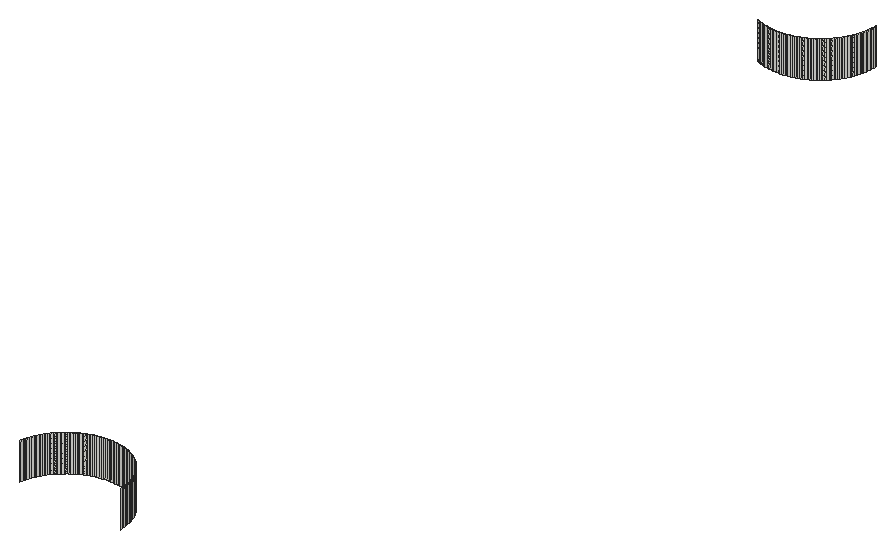
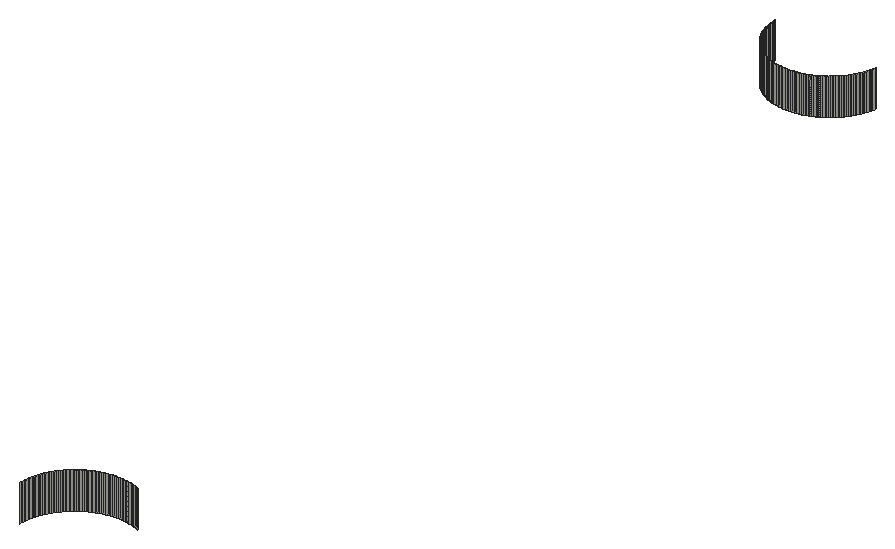
# SketchUp Ruby script. Lengths in inches.
U = 1.inch
M = Sketchup.active_model
def pt(a) = Geom::Point3d.new(a.map { |v| v * U })
def face(e, loops, mat)
  f = e.add_face(loops[0].map { |a| pt(a) })
  loops[1..].each { |l| e.add_face(l.map { |a| pt(a) }).erase! }
  f.material = f.back_material = mat if mat
  f
end
# faces: each face lists its corners as indices into pts; further lists are holes
def faces(e, pts, list, mat = nil) = list.each { |f| face(e, (f[0].is_a?(Array) ? f : [f]).map { |l| l.map { |i| pts[i] } }, mat) }
# xy, xz, yz: faces in a plane at the given z, y or x. An outline is a flat list of corners, or four numbers for a rectangle; further outlines are holes
def ring(l) = l.size == 4 ? [[l[0], l[1]], [l[2], l[1]], [l[2], l[3]], [l[0], l[3]]] : l.each_slice(2).to_a
def flat(e, list, mat, &to3) = list.each { |f| face(e, (f[0].is_a?(Array) ? f : [f]).map { |l| ring(l).map { |u, v| to3.(u, v) } }, mat) }
def xy(e, z, list, mat = nil) = flat(e, list, mat) { |x, y| [x, y, z] }
def xz(e, y, list, mat = nil) = flat(e, list, mat) { |x, z| [x, y, z] }
def yz(e, x, list, mat = nil) = flat(e, list, mat) { |y, z| [x, y, z] }
def lines(e, pts, list) = list.each { |a, b| e.add_line(pt(pts[a]), pt(pts[b])) }
# prism: a flat outline (further loops are holes) pulled along v
def prism(e, loops, v, mat = nil)
  f = face(e, loops, mat); d = Geom::Vector3d.new(v.map { |x| x * U })
  f.pushpull(f.normal.samedirection?(d) ? d.length : -d.length)
end
def box(e, o, s, mat = nil) = prism(e, [[o, [o[0] + s[0], o[1], o[2]], [o[0] + s[0], o[1] + s[1], o[2]], [o[0], o[1] + s[1], o[2]]]], [0, 0, s[2]], mat)
def at(x, y, z, deg = 0) = Geom::Transformation.translation(pt([x, y, z])) * Geom::Transformation.rotation(ORIGIN, Z_AXIS, deg.degrees)
def axes(o, x, y, z) = Geom::Transformation.new([*x, 0, *y, 0, *z, 0, *pt(o).to_a, 1])
def part(name) = M.definitions.add(name)
# library, detail: a bought-in or finely detailed component or shape, given as its bounding box
def library(name, o, s) = part(name).tap { |d| box(d.entities, o, s) }
def detail(e, o, s) = box(e.add_group.entities, o, s)
def put(e, d, t, mat = nil) = e.add_instance(d, t).tap { |i| i.material = mat if mat }
def group(e, t, mat = nil) = e.add_group.tap { |g| g.transformation = t; g.material = mat if mat }.entities
root = M.entities
xz(root,27,[[156.34,108,156.42,110],[156.42,108,156.5,110],[156.5,108,156.58,110],[156.58,108,156.66,110]])
xz(root,72.5,[[156.34,108,156.42,110],[156.42,108,156.5,110],[156.5,108,156.58,110],[156.58,108,156.66,110]])
yz(root,159.5,[[24,108,24.08,110],[24.08,108,24.16,110],[75.34,108,75.42,110],[75.42,108,75.5,110]])
p = [[159.48,24.3125,108],[159.49,24.24,108],[159.49,24.24,110],[159.48,24.3125,110],[159.5,24.16,108],[159.5,24.16,110],
  [159.47,24.39,108],[159.47,24.39,110],[159.46,24.47,108],[159.46,24.47,110],[153.55,24.55,108],[153.57,24.625,108],
  [153.57,24.625,110],[153.55,24.55,110],[159.43,24.625,108],[159.45,24.55,108],[159.45,24.55,110],[159.43,24.625,110],
  [153.58,24.7,108],[153.58,24.7,110],[159.42,24.7,108],[159.42,24.7,110],[153.6,24.78,108],[153.6,24.78,110],
  [159.4,24.78,108],[159.4,24.78,110],[153.625,24.85,108],[153.625,24.85,110],[159.375,24.85,108],[159.375,24.85,110],
  [153.65,24.93,108],[153.65,24.93,110],[153.67,25,108],[153.67,25,110],[159.33,25,108],[159.35,24.93,108],
  [159.35,24.93,110],[159.33,25,110],[153.7,25.08,108],[153.7,25.08,110],[159.3,25.08,108],[159.3,25.08,110],
  [153.73,25.15,108],[153.73,25.15,110],[153.76,25.22,108],[153.76,25.22,110],[159.24,25.22,108],[159.27,25.15,108],
  [159.27,25.15,110],[159.24,25.22,110],[153.79,25.29,108],[153.79,25.29,110],[159.21,25.29,108],[159.21,25.29,110],
  [153.83,25.36,108],[153.83,25.36,110],[159.17,25.36,108],[159.17,25.36,110],[153.86,25.43,108],[153.86,25.43,110],
  [153.9,25.5,108],[153.9,25.5,110],[159.1,25.5,108],[159.14,25.43,108],[159.14,25.43,110],[159.1,25.5,110],
  [153.94,25.57,108],[153.94,25.57,110],[159.06,25.57,108],[159.06,25.57,110],[153.98,25.63,108],[153.98,25.63,110],
  [154.03,25.7,108],[154.03,25.7,110],[158.97,25.7,108],[159.02,25.63,108],[159.02,25.63,110],[158.97,25.7,110],
  [154.07,25.76,108],[154.07,25.76,110],[158.93,25.76,108],[158.93,25.76,110],[154.12,25.83,108],[154.12,25.83,110],
  [154.17,25.89,108],[154.17,25.89,110],[158.83,25.89,108],[158.88,25.83,108],[158.88,25.83,110],[158.83,25.89,110],
  [154.22,25.95,108],[154.22,25.95,110],[154.27,26.01,108],[154.27,26.01,110],[158.73,26.01,108],[158.78,25.95,108],
  [158.78,25.95,110],[158.73,26.01,110],[154.32,26.07,108],[154.32,26.07,110],[158.68,26.07,108],[158.68,26.07,110],
  [154.38,26.12,108],[154.38,26.12,110],[154.43,26.18,108],[154.43,26.18,110],[158.57,26.18,108],[158.62,26.12,108],
  [158.62,26.12,110],[158.57,26.18,110],[154.49,26.23,108],[154.49,26.23,110],[154.55,26.28,108],[154.55,26.28,110],
  [158.45,26.28,108],[158.51,26.23,108],[158.51,26.23,110],[158.45,26.28,110],[154.61,26.33,108],[154.61,26.33,110],
  [154.67,26.38,108],[154.67,26.38,110],[158.33,26.38,108],[158.39,26.33,108],[158.39,26.33,110],[158.33,26.38,110],
  [154.74,26.43,108],[154.74,26.43,110],[154.8,26.47,108],[154.8,26.47,110],[158.2,26.47,108],[158.26,26.43,108],
  [158.26,26.43,110],[158.2,26.47,110],[154.87,26.52,108],[154.87,26.52,110],[154.93,26.56,108],[154.93,26.56,110],
  [158.07,26.56,108],[158.13,26.52,108],[158.13,26.52,110],[158.07,26.56,110],[155,26.6,108],[155,26.6,110],
  [155.07,26.64,108],[155.07,26.64,110],[155.14,26.67,108],[155.14,26.67,110],[157.86,26.67,108],[157.93,26.64,108],
  [157.93,26.64,110],[157.86,26.67,110],[158,26.6,108],[158,26.6,110],[155.21,26.71,108],[155.21,26.71,110],
  [155.28,26.74,108],[155.28,26.74,110],[155.35,26.77,108],[155.35,26.77,110],[157.65,26.77,108],[157.72,26.74,108],
  [157.72,26.74,110],[157.65,26.77,110],[157.79,26.71,108],[157.79,26.71,110],[155.42,26.8,108],[155.42,26.8,110],
  [155.5,26.83,108],[155.5,26.83,110],[155.57,26.85,108],[155.57,26.85,110],[157.43,26.85,108],[157.5,26.83,108],
  [157.5,26.83,110],[157.43,26.85,110],[157.58,26.8,108],[157.58,26.8,110],[155.65,26.875,108],[155.65,26.875,110],
  [155.72,26.9,108],[155.72,26.9,110],[155.8,26.92,108],[155.8,26.92,110],[155.875,26.93,108],[155.875,26.93,110],
  [155.95,26.95,108],[155.95,26.95,110],[156.03,26.96,108],[156.03,26.96,110],[156.97,26.96,108],[157.05,26.95,108],
  [157.05,26.95,110],[156.97,26.96,110],[157.125,26.93,108],[157.125,26.93,110],[157.2,26.92,108],[157.2,26.92,110],
  [157.28,26.9,108],[157.28,26.9,110],[157.35,26.875,108],[157.35,26.875,110],[156.11,26.97,108],[156.11,26.97,110],
  [156.1875,26.98,108],[156.1875,26.98,110],[156.26,26.99,108],[156.26,26.99,110],[156.34,27,108],[156.34,27,110],
  [156.66,27,108],[156.74,26.99,108],[156.74,26.99,110],[156.66,27,110],[156.8125,26.98,108],[156.8125,26.98,110],
  [156.89,26.97,108],[156.89,26.97,110],[156.11,72.53,108],[156.03,72.54,108],[156.03,72.54,110],[156.11,72.53,110],
  [155.95,72.55,108],[155.95,72.55,110],[156.1875,72.52,108],[156.1875,72.52,110],[156.26,72.51,108],[156.26,72.51,110],
  [156.34,72.5,108],[156.34,72.5,110],[156.8125,72.52,108],[156.74,72.51,108],[156.74,72.51,110],[156.8125,72.52,110],
  [156.66,72.5,108],[156.66,72.5,110],[156.89,72.53,108],[156.89,72.53,110],[156.97,72.54,108],[156.97,72.54,110],
  [157.05,72.55,108],[157.05,72.55,110],[155.57,72.65,108],[155.5,72.67,108],[155.5,72.67,110],[155.57,72.65,110],
  [155.72,72.6,108],[155.65,72.625,108],[155.65,72.625,110],[155.72,72.6,110],[155.8,72.58,108],[155.8,72.58,110],
  [155.875,72.57,108],[155.875,72.57,110],[157.125,72.57,108],[157.125,72.57,110],[157.2,72.58,108],[157.2,72.58,110],
  [157.28,72.6,108],[157.28,72.6,110],[157.35,72.625,108],[157.35,72.625,110],[157.5,72.67,108],[157.43,72.65,108],
  [157.43,72.65,110],[157.5,72.67,110],[155.35,72.73,108],[155.28,72.76,108],[155.28,72.76,110],[155.35,72.73,110],
  [155.42,72.7,108],[155.42,72.7,110],[157.58,72.7,108],[157.58,72.7,110],[157.72,72.76,108],[157.65,72.73,108],
  [157.65,72.73,110],[157.72,72.76,110],[157.79,72.79,108],[157.79,72.79,110],[157.86,72.83,108],[157.86,72.83,110],
  [157.93,72.86,108],[157.93,72.86,110],[158,72.9,108],[158,72.9,110],[158.07,72.94,108],[158.07,72.94,110],
  [158.13,72.98,108],[158.13,72.98,110],[158.2,73.03,108],[158.2,73.03,110],[158.26,73.07,108],[158.26,73.07,110],
  [158.39,73.17,108],[158.33,73.12,108],[158.33,73.12,110],[158.39,73.17,110],[158.51,73.27,108],[158.45,73.22,108],
  [158.45,73.22,110],[158.51,73.27,110],[158.57,73.32,108],[158.57,73.32,110],[158.62,73.38,108],[158.62,73.38,110],
  [158.68,73.43,108],[158.68,73.43,110],[158.73,73.49,108],[158.73,73.49,110],[158.78,73.55,108],[158.78,73.55,110],
  [158.88,73.67,108],[158.83,73.61,108],[158.83,73.61,110],[158.88,73.67,110],[158.97,73.8,108],[158.93,73.74,108],
  [158.93,73.74,110],[158.97,73.8,110],[159.02,73.87,108],[159.02,73.87,110],[159.06,73.93,108],[159.06,73.93,110],
  [159.1,74,108],[159.1,74,110],[159.14,74.07,108],[159.14,74.07,110],[159.17,74.14,108],[159.17,74.14,110],
  [159.21,74.21,108],[159.21,74.21,110],[159.24,74.28,108],[159.24,74.28,110],[159.27,74.35,108],[159.27,74.35,110],
  [159.33,74.5,108],[159.3,74.42,108],[159.3,74.42,110],[159.33,74.5,110],[159.35,74.57,108],[159.35,74.57,110],
  [159.4,74.72,108],[159.375,74.65,108],[159.375,74.65,110],[159.4,74.72,110],[159.42,74.8,108],[159.42,74.8,110],
  [159.43,74.875,108],[159.43,74.875,110],[159.45,74.95,108],[159.45,74.95,110],[159.46,75.03,108],[159.46,75.03,110],
  [159.47,75.11,108],[159.47,75.11,110],[159.48,75.1875,108],[159.48,75.1875,110],[159.49,75.26,108],[159.49,75.26,110],
  [159.5,75.34,108],[159.5,75.34,110]]
faces(root,p,[[0,1,2,3],[1,4,5,2],[6,0,3,7],[8,6,7,9],[10,11,12,13],[14,15,16,17],[15,8,9,16],[11,18,19,12],
  [20,14,17,21],[18,22,23,19],[24,20,21,25],[22,26,27,23],[28,24,25,29],[26,30,31,27],[30,32,33,31],[34,35,36,37],
  [35,28,29,36],[32,38,39,33],[40,34,37,41],[38,42,43,39],[42,44,45,43],[46,47,48,49],[47,40,41,48],[44,50,51,45],
  [52,46,49,53],[50,54,55,51],[56,52,53,57],[54,58,59,55],[58,60,61,59],[62,63,64,65],[63,56,57,64],[60,66,67,61],
  [68,62,65,69],[66,70,71,67],[70,72,73,71],[74,75,76,77],[75,68,69,76],[72,78,79,73],[80,74,77,81],[78,82,83,79],
  [82,84,85,83],[86,87,88,89],[87,80,81,88],[84,90,91,85],[90,92,93,91],[94,95,96,97],[95,86,89,96],[92,98,99,93],
  [100,94,97,101],[98,102,103,99],[102,104,105,103],[106,107,108,109],[107,100,101,108],[104,110,111,105],[110,112,113,111],[114,115,116,117],
  [115,106,109,116],[112,118,119,113],[118,120,121,119],[122,123,124,125],[123,114,117,124],[120,126,127,121],[126,128,129,127],[130,131,132,133],
  [131,122,125,132],[128,134,135,129],[134,136,137,135],[138,139,140,141],[139,130,133,140],[136,142,143,137],[142,144,145,143],[144,146,147,145],
  [148,149,150,151],[149,152,153,150],[152,138,141,153],[146,154,155,147],[154,156,157,155],[156,158,159,157],[160,161,162,163],[161,164,165,162],
  [164,148,151,165],[158,166,167,159],[166,168,169,167],[168,170,171,169],[172,173,174,175],[173,176,177,174],[176,160,163,177],[170,178,179,171],
  [178,180,181,179],[180,182,183,181],[182,184,185,183],[184,186,187,185],[186,188,189,187],[190,191,192,193],[191,194,195,192],[194,196,197,195],
  [196,198,199,197],[198,200,201,199],[200,172,175,201],[188,202,203,189],[202,204,205,203],[204,206,207,205],[206,208,209,207],[210,211,212,213],
  [211,214,215,212],[214,216,217,215],[216,190,193,217],[218,219,220,221],[219,222,223,220],[224,218,221,225],[226,224,225,227],[228,226,227,229],
  [230,231,232,233],[231,234,235,232],[236,230,233,237],[238,236,237,239],[240,238,239,241],[242,243,244,245],[246,247,248,249],[247,242,245,248],
  [250,246,249,251],[252,250,251,253],[222,252,253,223],[254,240,241,255],[256,254,255,257],[258,256,257,259],[260,258,259,261],[262,263,264,265],
  [263,260,261,264],[266,267,268,269],[243,270,271,244],[270,266,269,271],[272,262,265,273],[274,275,276,277],[275,272,273,276],[278,274,277,279],
  [280,278,279,281],[282,280,281,283],[284,282,283,285],[286,284,285,287],[288,286,287,289],[290,288,289,291],[292,290,291,293],[294,295,296,297],
  [295,292,293,296],[298,299,300,301],[299,294,297,300],[302,298,301,303],[304,302,303,305],[306,304,305,307],[308,306,307,309],[310,308,309,311],
  [312,313,314,315],[313,310,311,314],[316,317,318,319],[317,312,315,318],[320,316,319,321],[322,320,321,323],[324,322,323,325],[326,324,325,327],
  [328,326,327,329],[330,328,329,331],[332,330,331,333],[334,332,333,335],[336,337,338,339],[337,334,335,338],[340,336,339,341],[342,343,344,345],
  [343,340,341,344],[346,342,345,347],[348,346,347,349],[350,348,349,351],[352,350,351,353],[354,352,353,355],[356,354,355,357],[358,356,357,359],
  [360,358,359,361]])
